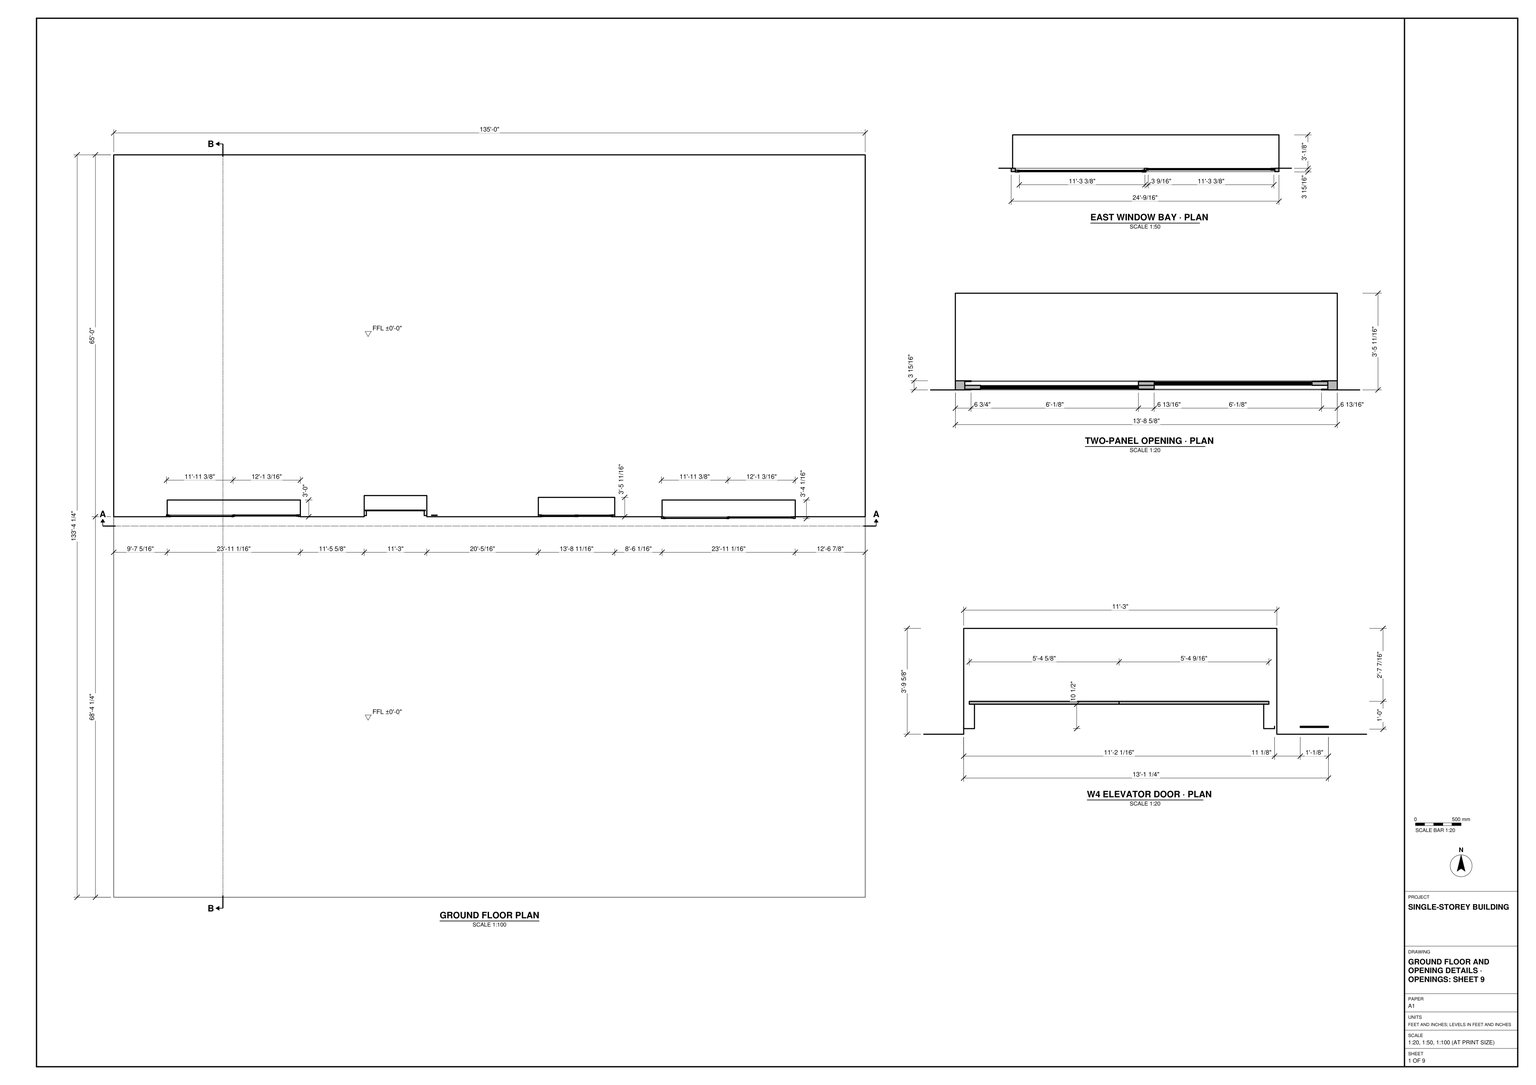
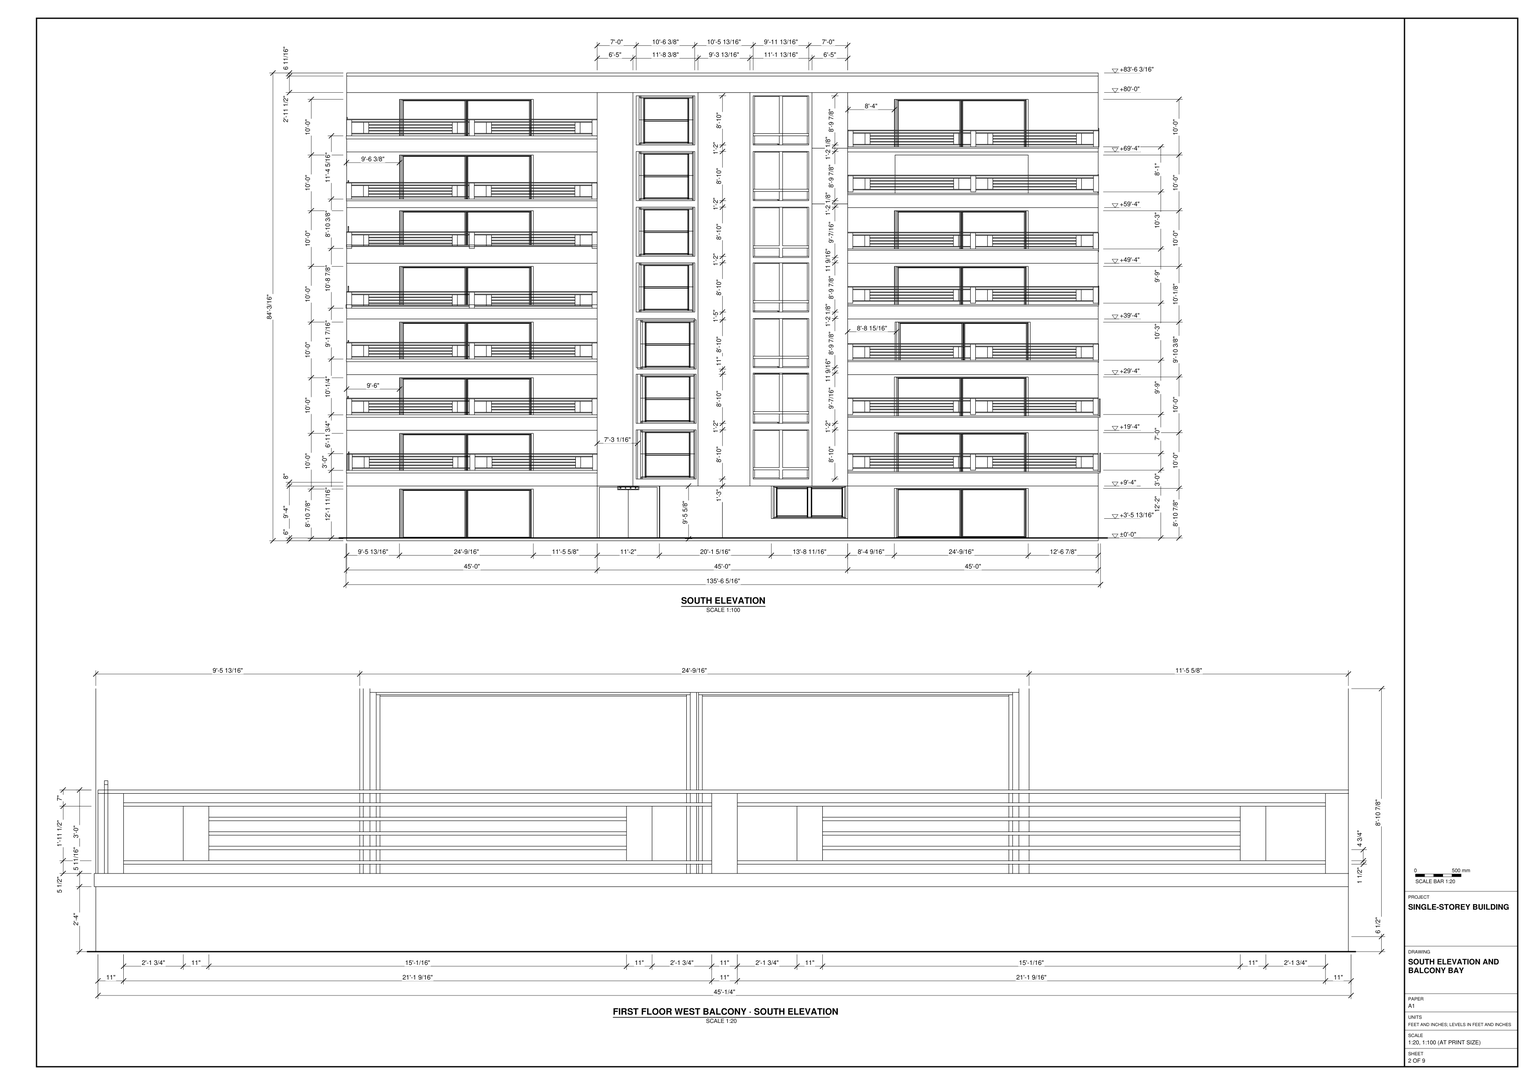
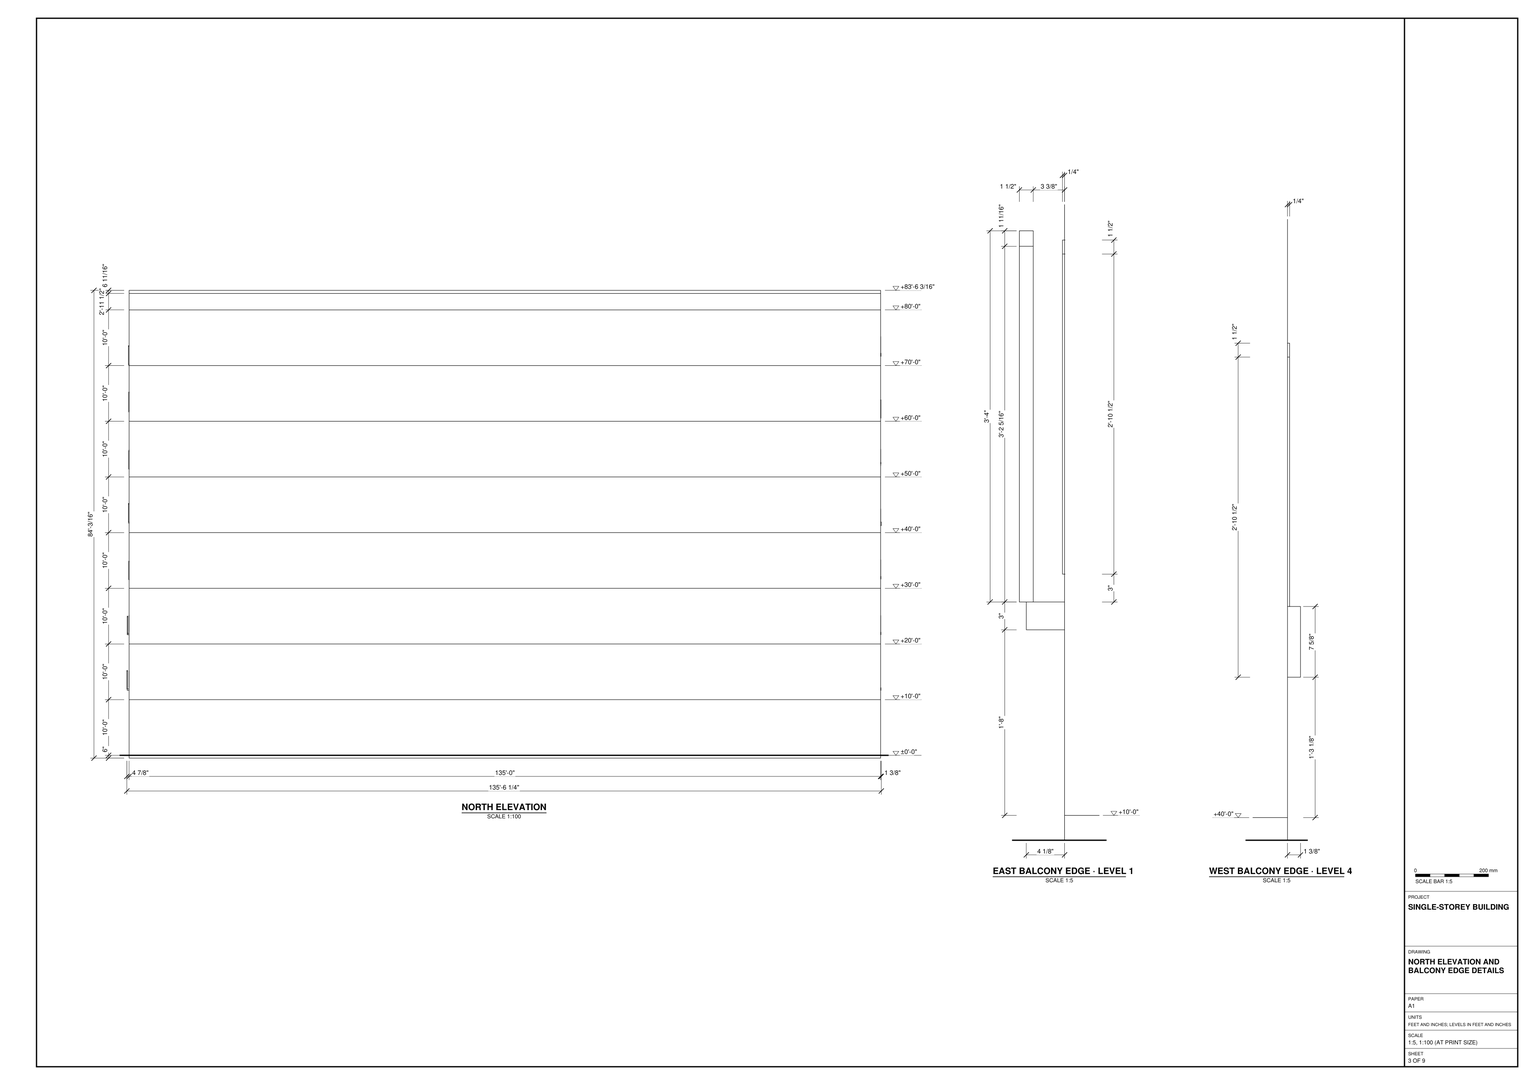
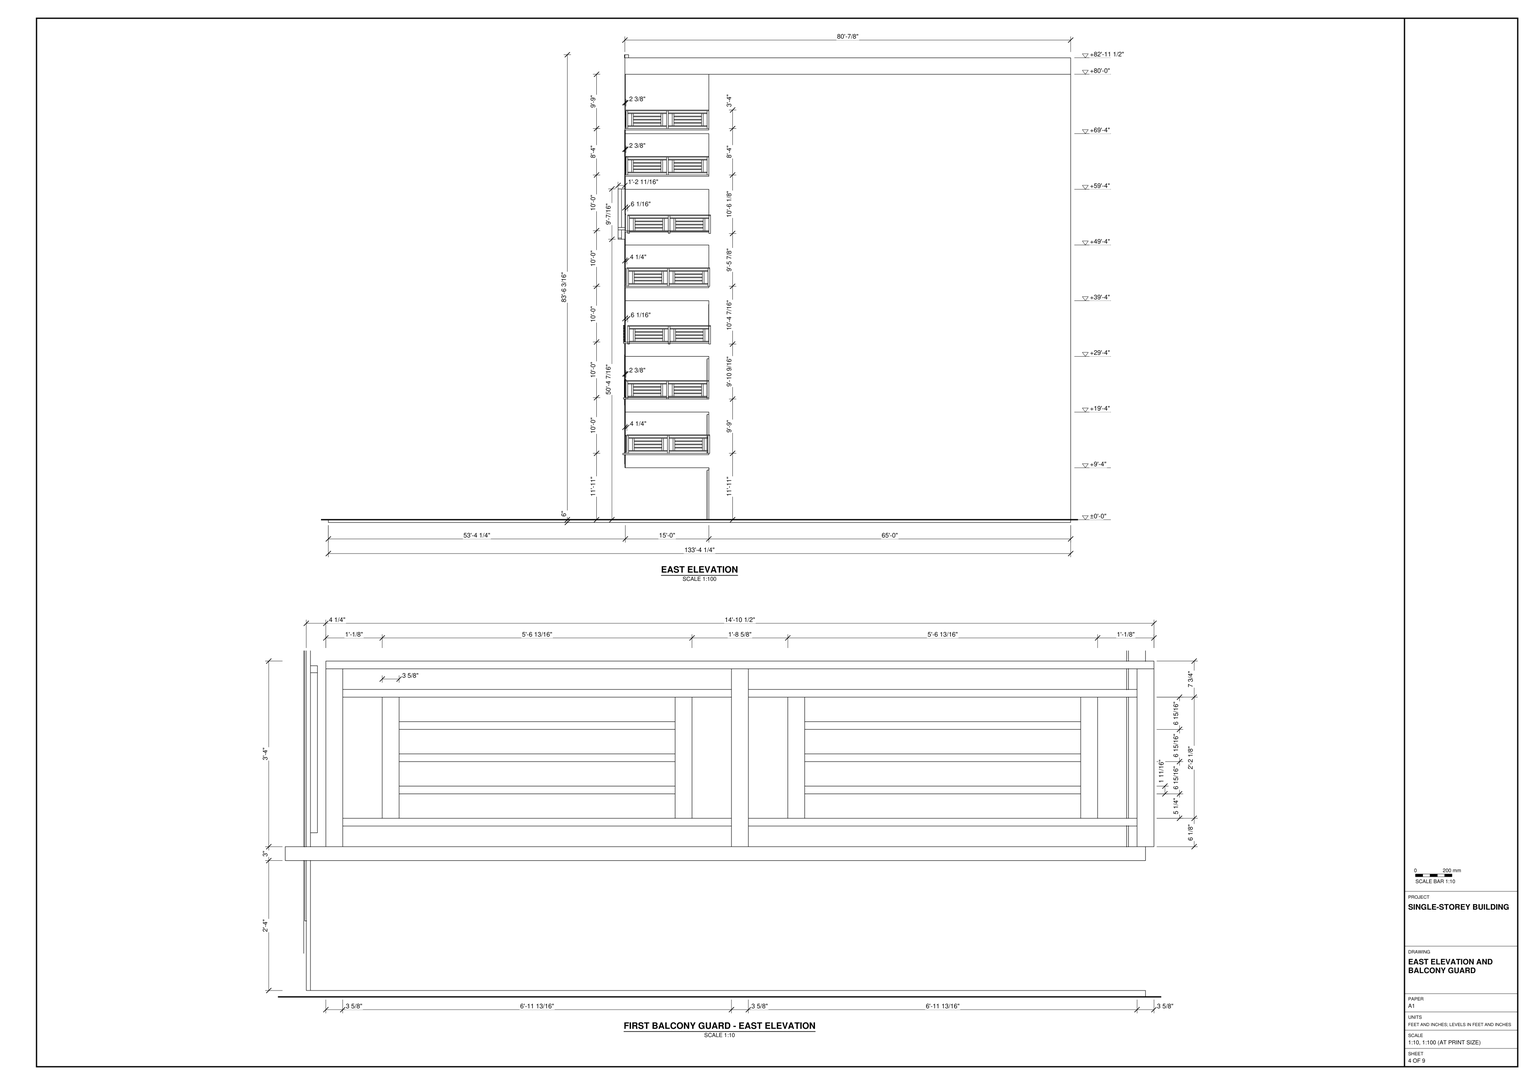
Build the building and its ground base in SketchUp from task_files/diagram_01.pdf. Work in feet and inches. Set the ground-floor finished level at ±0'-0". The overall model dimensions are 135'-6 1/4" along X, 133'-4 1/4" along Y and 84'-3/16" along Z. Use the plan to locate the south wall within the full depth of the base; the base continues south beyond the building.

Model the walls at the thicknesses drawn, with the floor slabs, balcony edges and flat roof following the elevations and sections. On the south face, place the wide outer openings behind the stacked balcony railings. Follow the balcony detail for the spacing of posts and horizontal rails. Keep the two narrower stacks of framed openings in the central bay distinct from the balcony bays. At ground level, use the opening plans to set the elevator door and the adjacent two-panel opening at their respective depths. Keep the north elevation plain, with the horizontal divisions shown.

Make shell elements such as walls, slabs and roof separate groups or components. Keep each furniture or joinery piece shown separate, and use components for repeated parts such as window units and railing sections. Any decor or loose items shown may use suitable library components. Save one SketchUp model as output_files/multi_storey_building_with_stacked_south_balconies.skp.

# SketchUp Ruby script. Lengths in inches.
U = 1.inch
M = Sketchup.active_model
def pt(a) = Geom::Point3d.new(a.map { |v| v * U })
def face(e, loops, mat)
  f = e.add_face(loops[0].map { |a| pt(a) })
  loops[1..].each { |l| e.add_face(l.map { |a| pt(a) }).erase! }
  f.material = f.back_material = mat if mat
  f
end
# faces: each face lists its corners as indices into pts; further lists are holes
def faces(e, pts, list, mat = nil) = list.each { |f| face(e, (f[0].is_a?(Array) ? f : [f]).map { |l| l.map { |i| pts[i] } }, mat) }
# xy, xz, yz: faces in a plane at the given z, y or x. An outline is a flat list of corners, or four numbers for a rectangle; further outlines are holes
def ring(l) = l.size == 4 ? [[l[0], l[1]], [l[2], l[1]], [l[2], l[3]], [l[0], l[3]]] : l.each_slice(2).to_a
def flat(e, list, mat, &to3) = list.each { |f| face(e, (f[0].is_a?(Array) ? f : [f]).map { |l| ring(l).map { |u, v| to3.(u, v) } }, mat) }
def xy(e, z, list, mat = nil) = flat(e, list, mat) { |x, y| [x, y, z] }
def xz(e, y, list, mat = nil) = flat(e, list, mat) { |x, z| [x, y, z] }
def yz(e, x, list, mat = nil) = flat(e, list, mat) { |y, z| [x, y, z] }
def lines(e, pts, list) = list.each { |a, b| e.add_line(pt(pts[a]), pt(pts[b])) }
# prism: a flat outline (further loops are holes) pulled along v
def prism(e, loops, v, mat = nil)
  f = face(e, loops, mat); d = Geom::Vector3d.new(v.map { |x| x * U })
  f.pushpull(f.normal.samedirection?(d) ? d.length : -d.length)
end
def box(e, o, s, mat = nil) = prism(e, [[o, [o[0] + s[0], o[1], o[2]], [o[0] + s[0], o[1] + s[1], o[2]], [o[0], o[1] + s[1], o[2]]]], [0, 0, s[2]], mat)
def at(x, y, z, deg = 0) = Geom::Transformation.translation(pt([x, y, z])) * Geom::Transformation.rotation(ORIGIN, Z_AXIS, deg.degrees)
def axes(o, x, y, z) = Geom::Transformation.new([*x, 0, *y, 0, *z, 0, *pt(o).to_a, 1])
def part(name) = M.definitions.add(name)
# library, detail: a bought-in or finely detailed component or shape, given as its bounding box
def library(name, o, s) = part(name).tap { |d| box(d.entities, o, s) }
def detail(e, o, s) = box(e.add_group.entities, o, s)
def put(e, d, t, mat = nil) = e.add_instance(d, t).tap { |i| i.material = mat if mat }
def group(e, t, mat = nil) = e.add_group.tap { |g| g.transformation = t; g.material = mat if mat }.entities
root = M.entities
M.materials.add("Glass_Tinted_Gray").color = [0, 0, 0]
M.materials["Glass_Tinted_Gray"].alpha = 0.125
M.materials.add("Painted Metal Railing").color = [35, 35, 35]
M.materials.add("[0043_SaddleBrown]").color = [139, 69, 19]
M.materials.add("[0047_Khaki]").color = [240, 230, 140]
M.materials.add("[0134_DimGray]").color = [105, 105, 105]
M.materials.add("[0135_DarkGray]").color = [81, 81, 81]
M.materials.add("[Mirror 02]").color = [229, 229, 229]
M.materials.add("[Terrazzo Light Blue]").color = [196, 214, 227]
c1 = library("Untitled",[0,0,0],[47.4375,3.75,63.125])
c2 = part("PENTEK_RP Fineline 50S_Sliding_DoorCase_E1")
box(c2.entities,[0,0,0],[1.51,3.66,99.27],"[0135_DarkGray]")
c3 = part("PENTEK_RP Fineline 50S_SlidingDooe_Case_E2")
box(c3.entities,[0,0,0],[96.25,3.66,1.51],"[0135_DarkGray]")
c4 = part("pentek_RP Fineline 50S_SlidingDoor_Case")
put(c4.entities,c2,at(97.76,0,0))
put(c4.entities,c3,at(1.51,0,0))
put(c4.entities,c2,at(0,0,0))
put(c4.entities,c3,at(1.51,0,97.76))
c5 = part("PENTEK_RP Fineline 50S_SlidingDoor_GlazingBead_2")
box(c5.entities,[0,0,0],[0.56,0.59,94.39],"[0135_DarkGray]")
c6 = part("PENTEK_RP Fineline 50S_SlidingDoor_Glass")
box(c6.entities,[0,0,0],[46.58,0.16,94.39],"Glass_Tinted_Gray")
c7 = part("PENTEK_RP Fineline 50S_SlidingDoor_GlazingBead")
box(c7.entities,[0,0,0],[45.47,0.59,0.56],"[0135_DarkGray]")
c8 = part("PENTEK_RP Fineline 50S_SlidingDoor_Leaf_E1")
xy(c8.entities,0,[[0,0,0.93,1.97],[0.93,1.57,1.49,1.97]],"[0135_DarkGray]")
xy(c8.entities,96.25,[[0,0,0.93,0,0.93,1.57,1.49,1.57,1.49,1.97,0,1.97]],"[0135_DarkGray]")
xz(c8.entities,0,[[0,0,0.93,96.25]],"[0135_DarkGray]")
xz(c8.entities,1.57,[[0.93,0,1.49,95.32],[0.93,95.32,1.49,96.25]],"[0135_DarkGray]")
xz(c8.entities,1.97,[[0,0,1.49,96.25]],"[0135_DarkGray]")
yz(c8.entities,0,[[0,0,1.97,96.25]],"[0135_DarkGray]")
yz(c8.entities,0.93,[[0,0,1.57,0.93],[0,0.93,1.57,95.32],[0,95.32,1.57,96.25]],"[0135_DarkGray]")
yz(c8.entities,1.49,[[1.57,0,1.97,95.32],[1.57,95.32,1.97,96.25]],"[0135_DarkGray]")
c9 = part("PENTEK_RP Fineline 50S_SlidingDoor_Leaf_E2")
xy(c9.entities,0,[[0,0,0,1.57,0.56,1.57,0.56,1.97,46.02,1.97,46.02,1.57,46.58,1.57,46.58,0]],"[0135_DarkGray]")
xy(c9.entities,0.93,[[0,0,46.58,1.57]],"[0135_DarkGray]")
xy(c9.entities,1.49,[[0.56,1.57,46.02,1.97]],"[0135_DarkGray]")
xz(c9.entities,0,[[0,0,46.58,0.93]],"[0135_DarkGray]")
xz(c9.entities,1.57,[[0,0,0.56,0.93],[46.02,0,46.58,0.93],[0.56,0.93,46.02,1.49]],"[0135_DarkGray]")
xz(c9.entities,1.97,[[0.56,0,46.02,1.49]],"[0135_DarkGray]")
yz(c9.entities,0,[[0,0,1.57,0.93]],"[0135_DarkGray]")
yz(c9.entities,0.56,[[1.57,0,1.97,0.93],[1.57,0.93,1.97,1.49]],"[0135_DarkGray]")
yz(c9.entities,46.02,[[1.57,0,1.97,0.93],[1.57,0.93,1.97,1.49]],"[0135_DarkGray]")
yz(c9.entities,46.58,[[0,0,1.57,0.93]],"[0135_DarkGray]")
c10 = part("PENTEK_RP Fineline S_SlidingDoor_Leaf1")
put(c10.entities,c5,at(0.93,0,0.93))
put(c10.entities,c5,at(46.96,0,0.93))
put(c10.entities,c6,at(1.49,1.42,0.93))
put(c10.entities,c7,at(1.49,0,0.93))
put(c10.entities,c6,at(1.49,0.59,0.93),"[Terrazzo Light Blue]")
put(c10.entities,c8,at(0,0,0))
put(c10.entities,c8,axes([48.44,0,0],[-1,0,0],[0,1,0],[0,0,1]))
put(c10.entities,c9,axes([0.93,0,96.25],[1,0,0],[0,1,0],[0,0,-1]))
put(c10.entities,c9,at(0.93,0,0))
put(c10.entities,c7,at(1.49,0,94.77))
c11 = part("PENTEK_RP Fineline 50S_SlidingDoor_Leaf2")
put(c11.entities,c6,at(1.49,1.42,0.93))
put(c11.entities,c7,at(1.49,0,94.77))
put(c11.entities,c5,at(46.96,0,0.93))
put(c11.entities,c6,at(1.49,0.59,0.93),"[Mirror 02]")
put(c11.entities,c5,at(0.93,0,0.93))
put(c11.entities,c8,at(0,0,0))
put(c11.entities,c8,axes([48.44,0,0],[-1,0,0],[0,1,0],[0,0,1]))
put(c11.entities,c7,at(1.49,0,0.93))
put(c11.entities,c9,axes([0.93,0,96.25],[1,0,0],[0,1,0],[0,0,-1]))
put(c11.entities,c9,at(0.93,0,0))
c12 = part("PENTEK - Slimmest Steel Sliding Door / Window\#1")
put(c12.entities,c4,at(0,-1.88,-0.09))
put(c12.entities,c10,at(1.51,-2.27,1.42))
put(c12.entities,c11,at(49.32,-0.3,1.42))
c13 = library("Elevator_Door[140]",[-13.125,-2.71,-1.46],[68.625,12,93.74])
c14 = part("Post")
box(c14.entities,[-0.75,-0.75,0],[1.5,1.5,34.5],"Painted Metal Railing")
c15 = part("Group43\#1")
box(c15.entities,[-0.75,0,0],[1.5,73.5,1.5],"Painted Metal Railing")
c16 = part("Group46\#1")
box(c16.entities,[-0.75,0.75,0],[1.5,34.5,1.5],"Painted Metal Railing")
c17 = part("Group49\#1")
box(c17.entities,[-0.75,0.75,0],[1.5,34.5,1.5],"Painted Metal Railing")
c18 = part("Group52\#1")
box(c18.entities,[-0.75,0.75,0],[1.5,34.5,1.5],"Painted Metal Railing")
c19 = part("Group55\#1")
box(c19.entities,[-0.75,0.75,0],[1.5,34.5,1.5],"Painted Metal Railing")
c20 = part("Inner Post")
box(c20.entities,[-0.75,-0.75,0],[1.5,1.5,23.5],"Painted Metal Railing")
c21 = part("Group59\#1")
box(c21.entities,[-0.75,0.75,0],[1.5,24.5,1.5],"Painted Metal Railing")
c22 = part("Group62\#1")
box(c22.entities,[-0.75,0.75,0],[1.5,24.5,1.5],"Painted Metal Railing")
c23 = part("Group65\#1")
box(c23.entities,[-0.75,0.75,0],[1.5,24.5,1.5],"Painted Metal Railing")
c24 = part("Inner Posts and Rails\#2")
put(c24.entities,c20,at(0,0,0,90))
put(c24.entities,c20,at(0,26,0,90))
put(c24.entities,c21,at(0,0,4.75))
put(c24.entities,c22,at(0,0,11))
put(c24.entities,c23,at(0,0,17.25))
c25 = part("Group69\#1")
box(c25.entities,[-0.75,0.75,0],[1.5,24.5,1.5],"Painted Metal Railing")
c26 = part("Group72\#1")
box(c26.entities,[-0.75,0.75,0],[1.5,24.5,1.5],"Painted Metal Railing")
c27 = part("Group75\#1")
box(c27.entities,[-0.75,0.75,0],[1.5,24.5,1.5],"Painted Metal Railing")
c28 = part("Inner Posts and Rails\#3")
put(c28.entities,c20,at(0,0,0,90))
put(c28.entities,c20,at(0,26,0,90))
put(c28.entities,c25,at(0,0,4.75))
put(c28.entities,c26,at(0,0,11))
put(c28.entities,c27,at(0,0,17.25))
c29 = part("Railing Assembly 14\#1")
put(c29.entities,c14,at(0,0,0))
put(c29.entities,c14,at(36,0,0))
put(c29.entities,c14,at(72,0,0))
put(c29.entities,c15,at(-0.75,0,34.5,-90))
put(c29.entities,c16,at(0,0,4,-90))
put(c29.entities,c17,at(36,0,4,-90))
put(c29.entities,c18,at(0,0,29,-90))
put(c29.entities,c19,at(36,0,29,-90))
put(c29.entities,c24,at(5,0,5.5,-90))
put(c29.entities,c28,at(41,0,5.5,-90))
c30 = part("Railing Assembly 14\#2")
put(c30.entities,c14,at(0,0,0))
put(c30.entities,c14,at(36,0,0))
put(c30.entities,c14,at(72,0,0))
put(c30.entities,c15,at(-0.75,0,34.5,-90))
put(c30.entities,c16,at(0,0,4,-90))
put(c30.entities,c17,at(36,0,4,-90))
put(c30.entities,c18,at(0,0,29,-90))
put(c30.entities,c19,at(36,0,29,-90))
put(c30.entities,c24,at(5,0,5.5,-90))
put(c30.entities,c28,at(41,0,5.5,-90))
c31 = library("Group\#21",[0,0,0],[47.24,3.9375,39.37])
c32 = library("Group\#22",[0,0,0],[23.62,3.9375,39.37])
xy(root,-6,[[1.4,0,1621.4,1600.25]])
xy(root,0,[[1.4,0,1621.4,0,1621.4,820.25,1470.54,820.25,1470.54,856.25,1183.49,856.25,1183.49,820.25,676.4,820.25,676.4,865.875,541.4,865.875,541.4,820.25,403.75,820.25,403.75,856.25,116.7,856.25,116.7,820.25,1.4,820.25],[1.4,820.25,116.7,820.25,116.7,856.25,403.75,856.25,403.75,820.25,541.4,820.25,541.4,865.875,676.4,865.875,676.4,820.25,1183.49,820.25,1183.49,856.25,1470.54,856.25,1470.54,820.25,1621.4,820.25,1621.4,1600.25,1.4,1600.25]])
xy(root,41.8125,[[916.73,820.25,1081.4,861.9375]])
xy(root,105.375,[[116.7,820.25,403.75,856.25],[1183.49,820.25,1470.54,856.25]])
xy(root,112,[[618.42,639.35,618.42,640.25,1.4,640.25,1.4,820.25,541.4,820.25,541.4,865.875,676.4,865.875,676.4,820.25,916.73,820.25,916.73,861.9375,1081.4,861.9375,1081.4,820.25,1621.4,820.25,1621.4,640.25,1004.4,640.25,1004.4,639.35,870.61,639.35,870.61,640.25,870.58,640.25,870.58,642.9375,758.8,642.9375,758.8,639.35]])
xy(root,120,[[870.58,639.35,870.61,640.25],[7.4,646.25,541.4,646.25,541.4,820.25,403.75,820.25,403.75,856.25,116.7,856.25,116.7,820.25,7.4,820.25],[1081.4,648.25,1613.4,648.25,1613.4,820.25,1470.54,820.25,1470.54,856.25,1183.49,856.25,1183.49,820.25,1081.4,820.25]])
xy(root,127,[[625.42,639.35,751.8,651.25],[877.58,639.35,997.4,651.25]])
xy(root,140,[[1081.4,634.8125,1621.4,640.25],[1621.4,634.8125,1625.52,820.25],[0.7,639.55,541.4,640.25],[0.7,640.25,1.4,820.25],[1.4,640.25,1.4,820.25,7.4,820.25,7.4,646.25,541.4,646.25,541.4,640.25],
  [1081.4,640.25,1081.4,648.25,1613.4,648.25,1613.4,820.25,1621.4,820.25,1621.4,640.25]])
xy(root,143,[[1081.4,634.8125,1625.52,634.8125,1625.52,820.25,1613.4,820.25,1613.4,648.25,1081.4,648.25]])
xy(root,145.6875,[[0.7,639.55,541.4,639.55,541.4,646.25,7.4,646.25,7.4,820.25,0.7,820.25]])
xy(root,225.375,[[116.7,820.25,403.75,856.25],[1183.49,820.25,1470.54,856.25]])
xy(root,232,[[1.4,640.25,541.4,820.25],[1081.4,640.25,1621.4,820.25]])
xy(root,233,[[625.42,639.35,751.8,651.25],[877.58,639.35,997.4,651.25]])
xy(root,240,[[7.4,646.25,541.4,646.25,541.4,820.25,403.75,820.25,403.75,856.25,116.7,856.25,116.7,820.25,7.4,820.25],[1081.4,648.25,1613.4,648.25,1613.4,820.25,1470.54,820.25,1470.54,856.25,1183.49,856.25,1183.49,820.25,1081.4,820.25]])
xy(root,247,[[625.42,639.35,751.8,651.25],[877.58,639.35,997.4,651.25]])
xy(root,260,[[1081.4,636.125,1621.4,640.25],[1621.4,636.125,1625.52,820.25],[0.7,639.55,1.4,820.25],[1.4,639.55,541.4,640.25],[1.4,640.25,1.4,820.25,7.4,820.25,7.4,646.25,541.4,646.25,541.4,640.25],
  [1081.4,640.25,1081.4,648.25,1613.4,648.25,1613.4,820.25,1621.4,820.25,1621.4,640.25]])
xy(root,263,[[1081.4,636.125,1625.52,636.125,1625.52,820.25,1613.4,820.25,1613.4,648.25,1081.4,648.25]])
xy(root,265.4375,[[0.7,639.55,541.4,639.55,541.4,646.25,7.4,646.25,7.4,820.25,0.7,820.25]])
xy(root,345.375,[[116.7,820.25,403.75,856.25],[1183.49,820.25,1470.54,856.25]])
xy(root,352,[[1.4,640.25,541.4,820.25],[1081.4,640.25,1621.4,820.25]])
xy(root,353,[[625.42,639.35,751.8,651.25],[877.58,639.35,997.4,651.25]])
xy(root,360,[[7.4,646.25,541.4,646.25,541.4,820.25,403.75,820.25,403.75,856.25,116.7,856.25,116.7,820.25,7.4,820.25],[1081.4,648.25,1613.4,648.25,1613.4,820.25,1470.54,820.25,1470.54,856.25,1183.49,856.25,1183.49,820.25,1081.4,820.25]])
xy(root,367,[[625.42,639.35,751.8,651.25],[877.58,639.35,997.4,651.25]])
xy(root,380,[[1081.4,636.125,1621.4,640.25],[1621.4,636.125,1622.2,820.25],[0.7,639.55,541.4,640.25],[0.7,640.25,1.4,820.25],[1.4,640.25,1.4,820.25,7.4,820.25,7.4,646.25,541.4,646.25,541.4,640.25],
  [1081.4,640.25,1081.4,648.25,1613.4,648.25,1613.4,820.25,1621.4,820.25,1621.4,640.25]])
xy(root,383,[[1081.4,636.125,1622.2,636.125,1622.2,820.25,1613.4,820.25,1613.4,648.25,1081.4,648.25]])
xy(root,385.6875,[[0.7,639.55,541.4,639.55,541.4,646.25,7.4,646.25,7.4,820.25,0.7,820.25]])
xy(root,465.375,[[116.7,820.25,403.75,856.25],[1183.49,820.25,1470.54,856.25]])
xy(root,472,[[1.4,640.25,541.4,820.25],[1081.4,640.25,1621.4,820.25]])
xy(root,473,[[625.42,639.35,751.8,651.25],[877.58,639.35,997.4,651.25]])
xy(root,480,[[7.4,646.25,541.4,646.25,541.4,820.25,403.75,820.25,403.75,856.25,116.7,856.25,116.7,820.25,7.4,820.25],[1081.4,648.25,1613.4,648.25,1613.4,820.25,1470.54,820.25,1470.54,856.25,1183.49,856.25,1183.49,820.25,1081.4,820.25]])
xy(root,487,[[625.42,639.35,751.8,651.25],[877.58,639.35,997.4,651.25]])
xy(root,495.125,[[0,638.85,541.4,640.25],[0,640.25,1.4,820.25],[1.4,640.25,1.4,820.25,7.4,820.25,7.4,646.25,541.4,646.25,541.4,640.25]])
xy(root,500,[[1081.4,639.45,1621.4,640.25],[1621.4,639.45,1622.2,820.25],[1081.4,640.25,1081.4,648.25,1613.4,648.25,1613.4,820.25,1621.4,820.25,1621.4,640.25]])
xy(root,502.75,[[0,638.85,541.4,638.85,541.4,646.25,7.4,646.25,7.4,820.25,0,820.25]])
xy(root,503,[[1081.4,639.45,1622.2,639.45,1622.2,820.25,1613.4,820.25,1613.4,648.25,1081.4,648.25]])
xy(root,585.375,[[116.7,820.25,403.75,856.25],[1183.49,820.25,1470.54,856.25]])
xy(root,592,[[1.4,640.25,541.4,820.25],[1081.4,640.25,1621.4,820.25]])
xy(root,593,[[625.42,639.35,751.8,651.25],[877.58,639.35,997.4,651.25]])
xy(root,600,[[7.4,646.25,541.4,646.25,541.4,820.25,403.75,820.25,403.75,856.25,116.7,856.25,116.7,820.25,7.4,820.25],[1081.4,648.25,1613.4,648.25,1613.4,820.25,1470.54,820.25,1470.54,856.25,1183.49,856.25,1183.49,820.25,1081.4,820.25]])
xy(root,607,[[625.42,639.35,751.8,651.25],[877.58,639.35,997.4,651.25]])
xy(root,620,[[1081.4,639.45,1621.4,640.25],[1621.4,639.45,1622.2,820.25],[1081.4,640.25,1081.4,648.25,1613.4,648.25,1613.4,820.25,1621.4,820.25,1621.4,640.25]])
xy(root,623,[[1081.4,639.45,1622.2,639.45,1622.2,820.25,1613.4,820.25,1613.4,648.25,1081.4,648.25]])
xy(root,628,[[0.7,639.55,541.4,640.25],[0.7,640.25,1.4,820.25],[1.4,640.25,1.4,820.25,7.4,820.25,7.4,646.25,541.4,646.25,541.4,640.25]])
xy(root,631.625,[[0.7,639.55,541.4,639.55,541.4,646.25,7.4,646.25,7.4,820.25,0.7,820.25]])
xy(root,705.375,[[116.7,820.25,403.75,856.25],[1183.49,820.25,1470.54,856.25]])
xy(root,712,[[1.4,640.25,541.4,820.25],[1081.4,640.25,1621.4,820.25]])
xy(root,713,[[625.42,639.35,751.8,651.25],[877.58,639.35,997.4,651.25]])
xy(root,720,[[7.4,646.25,541.4,646.25,541.4,820.25,403.75,820.25,403.75,856.25,116.7,856.25,116.7,820.25,7.4,820.25],[1081.4,648.25,1613.4,648.25,1613.4,820.25,1470.54,820.25,1470.54,856.25,1183.49,856.25,1183.49,820.25,1081.4,820.25]])
xy(root,726.6875,[[0.8,639.65,541.4,640.25],[0.8,640.25,1.4,820.25],[1.4,640.25,1.4,820.25,7.4,820.25,7.4,646.25,541.4,646.25,541.4,640.25]])
xy(root,727,[[625.42,639.35,751.8,651.25],[877.58,639.35,997.4,651.25]])
xy(root,730.375,[[0.8,639.65,541.4,639.65,541.4,646.25,7.4,646.25,7.4,820.25,0.8,820.25]],"[0043_SaddleBrown]")
xy(root,740,[[1081.4,639.45,1621.4,640.25],[1621.4,639.45,1622.2,820.25],[1081.4,640.25,1081.4,648.25,1613.4,648.25,1613.4,820.25,1621.4,820.25,1621.4,640.25]])
xy(root,743,[[1081.4,639.45,1622.2,639.45,1622.2,820.25,1613.4,820.25,1613.4,648.25,1081.4,648.25]])
xy(root,825.375,[[116.7,820.25,403.75,856.25],[1183.49,820.25,1470.54,856.25]])
xy(root,832,[[1.4,640.25,541.4,820.25],[1081.4,640.25,1621.4,820.25]])
xy(root,833,[[625.42,639.35,751.8,651.25],[877.58,639.35,997.4,651.25]])
xy(root,840,[[1081.4,639.45,1621.4,640.25],[1621.4,639.45,1622.2,820.25],[1081.4,640.25,1081.4,648.25,1613.4,648.25,1613.4,820.25,1621.4,820.25,1621.4,640.25],[7.4,646.25,541.4,646.25,541.4,820.25,403.75,820.25,403.75,856.25,116.7,856.25,116.7,820.25,7.4,820.25],[1081.4,648.25,1613.4,648.25,1613.4,820.25,1470.54,820.25,1470.54,856.25,1183.49,856.25,1183.49,820.25,1081.4,820.25]])
xy(root,843,[[1081.4,639.45,1622.2,639.45,1622.2,820.25,1613.4,820.25,1613.4,648.25,1081.4,648.25]])
xy(root,847,[[625.42,639.35,751.8,651.25],[877.58,639.35,997.4,651.25]])
xy(root,860,[[0.6,639.45,1.4,640.25],[1.4,639.45,541.4,640.25],[0.6,640.25,1.4,820.25],[1.4,640.25,1.4,820.25,7.4,820.25,7.4,646.25,541.4,646.25,541.4,640.25]])
xy(root,866.6875,[[0.6,639.45,541.4,639.45,541.4,646.25,7.4,646.25,7.4,820.25,0.6,820.25]])
xy(root,945.375,[[116.7,820.25,403.75,856.25],[1183.49,820.25,1470.54,856.25]])
xy(root,953,[[625.42,639.35,751.8,651.25],[877.58,639.35,997.4,651.25]])
xy(root,960,[[1.4,639.35,541.4,820.25],[618.42,639.35,618.42,640.25,541.4,640.25,541.4,820.25,1.4,820.25,1.4,1600.25,1621.4,1600.25,1621.4,820.25,1081.4,820.25,1081.4,640.25,1004.4,640.25,1004.4,639.35,870.58,639.35,870.58,642.9375,758.8,642.9375,758.8,639.35],[541.4,639.35,618.42,640.25],[758.8,639.35,870.58,642.9375],[1004.4,639.35,1081.4,640.25],
  [1081.4,639.35,1621.4,820.25]])
xy(root,995.5,[[1.4,639.35,1621.4,647.35],[1.4,647.35,1621.4,1600.25]])
xy(root,995.5,[[1.4,638.45,1621.4,639.35]],"[0043_SaddleBrown]")
xy(root,1002.1875,[[1.4,638.45,1621.4,647.35]])
xz(root,0,[[1.4,-6,1621.4,0]])
xz(root,634.8125,[[1081.4,140,1625.52,143]])
xz(root,636.125,[[1081.4,260,1625.52,263],[1081.4,380,1622.2,383]])
xz(root,638.45,[[1.4,995.5,1621.4,1002.1875]],"[0043_SaddleBrown]")
xz(root,638.85,[[0,495.125,541.4,502.75]],"[0043_SaddleBrown]")
xz(root,639.35,[[1.4,960,1621.4,995.5]])
xz(root,639.35,[[[618.42,112,758.8,960],[625.42,847,751.8,953],[625.42,607,751.8,713],[625.42,367,751.8,473],[625.42,127,751.8,233],[625.42,247,751.8,353],[625.42,487,751.8,593],[625.42,727,751.8,833]],[[870.61,112,1004.4,112,1004.4,960,870.58,960,870.58,120,870.61,120],[877.58,247,997.4,353],[877.58,847,997.4,953],[877.58,607,997.4,713],[877.58,127,997.4,233],[877.58,487,997.4,593],[877.58,727,997.4,833],[877.58,367,997.4,473]]],"[0134_DimGray]")
xz(root,639.45,[[1081.4,500,1622.2,503],[1081.4,620,1622.2,623],[1081.4,740,1622.2,743],[1081.4,840,1622.2,843],[0.6,860,541.4,866.6875]])
xz(root,639.55,[[0.7,140,541.4,145.6875]])
xz(root,639.55,[[0.7,260,541.4,265.4375],[0.7,380,541.4,385.6875],[0.7,628,541.4,631.625]],"[0043_SaddleBrown]")
xz(root,639.65,[[0.8,726.6875,541.4,730.375]],"[0043_SaddleBrown]")
xz(root,640.25,[[1.4,112,541.4,140],[870.58,112,870.61,120],[1081.4,112,1621.4,140],[1.4,232,541.4,260],[1081.4,232,1621.4,260],
  [1.4,352,541.4,380],[1081.4,352,1621.4,380],[1.4,472,541.4,495.125],[1081.4,472,1621.4,500],[1.4,592,541.4,628],
  [1081.4,592,1621.4,620],[1.4,712,541.4,726.6875],[1081.4,712,1621.4,740],[1.4,832,541.4,860],[1081.4,832,1621.4,840]])
xz(root,640.25,[[541.4,112,618.42,960],[1004.4,112,1081.4,720],[1004.4,720,1081.4,840],[1004.4,840,1081.4,960]],"[0134_DimGray]")
xz(root,642.9375,[[758.8,112,870.58,960]],"[0134_DimGray]")
xz(root,646.25,[[7.4,120,541.4,140],[7.4,140,541.4,145.6875],[7.4,240,541.4,260],[7.4,260,541.4,265.4375],[7.4,360,541.4,380],
  [7.4,380,541.4,385.6875],[7.4,480,541.4,495.125],[7.4,495.125,541.4,502.75],[7.4,600,541.4,628],[7.4,628,541.4,631.625],
  [7.4,720,541.4,726.6875],[7.4,726.6875,541.4,730.375],[7.4,840,541.4,860],[7.4,860,541.4,866.6875]])
xz(root,647.35,[[1.4,995.5,1621.4,1002.1875]])
xz(root,648.25,[[1081.4,120,1613.4,140],[1081.4,140,1613.4,143],[1081.4,240,1613.4,260],[1081.4,260,1613.4,263],[1081.4,360,1613.4,380],
  [1081.4,380,1613.4,383],[1081.4,480,1613.4,500],[1081.4,500,1613.4,503],[1081.4,600,1613.4,620],[1081.4,620,1613.4,623],
  [1081.4,720,1613.4,740],[1081.4,740,1613.4,743],[1081.4,840,1613.4,843]])
xz(root,651.25,[[625.42,127,751.8,233],[877.58,127,997.4,233],[625.42,247,751.8,353],[877.58,247,997.4,353],[625.42,367,751.8,473],
  [877.58,367,997.4,473],[625.42,487,751.8,593],[877.58,487,997.4,593],[625.42,607,751.8,713],[877.58,607,997.4,713],
  [625.42,727,751.8,833],[877.58,727,997.4,833],[625.42,847,751.8,953],[877.58,847,997.4,953]])
xz(root,820.25,[[0.7,140,1.4,145.6875],[1.4,140,7.4,145.6875],[1613.4,140,1621.4,143],[1621.4,140,1625.52,143],[0.7,260,1.4,265.4375],
  [1.4,260,7.4,265.4375],[1613.4,260,1621.4,263],[1621.4,260,1625.52,263],[1.4,360,7.4,380],[0.7,380,1.4,385.6875],
  [1.4,380,7.4,385.6875],[1613.4,380,1621.4,383],[1621.4,380,1622.2,383],[0,495.125,1.4,502.75],[1.4,495.125,7.4,502.75],
  [1613.4,500,1621.4,503],[1621.4,500,1622.2,503],[1613.4,620,1621.4,623],[1621.4,620,1622.2,623],[0.7,628,1.4,631.625],
  [1.4,628,7.4,631.625],[1.4,720,7.4,726.6875],[0.8,726.6875,1.4,730.375],[1.4,726.6875,7.4,730.375],[1613.4,740,1621.4,743],
  [1621.4,740,1622.2,743],[1613.4,840,1621.4,843],[1621.4,840,1622.2,843],[0.6,860,1.4,866.6875],[1.4,860,7.4,866.6875]])
xz(root,820.25,[[1.4,0,116.7,0,116.7,105.375,403.75,105.375,403.75,0,541.4,0,541.4,112,1.4,112],[676.4,0,811.4,112],[811.4,0,1081.4,0,1081.4,41.8125,916.73,41.8125,916.73,112,811.4,112],[1081.4,0,1183.49,0,1183.49,105.375,1470.54,105.375,1470.54,0,1621.4,0,1621.4,112,1081.4,112],[7.4,120,116.7,120,116.7,225.375,403.75,225.375,403.75,120,541.4,120,541.4,232,1.4,232,1.4,145.6875,7.4,145.6875],
  [1081.4,120,1183.49,120,1183.49,225.375,1470.54,225.375,1470.54,120,1613.4,120,1613.4,143,1621.4,143,1621.4,232,1081.4,232],[7.4,240,116.7,240,116.7,345.375,403.75,345.375,403.75,240,541.4,240,541.4,352,1.4,352,1.4,265.4375,7.4,265.4375],[1081.4,240,1183.49,240,1183.49,345.375,1470.54,345.375,1470.54,240,1613.4,240,1613.4,263,1621.4,263,1621.4,352,1081.4,352],[7.4,360,116.7,360,116.7,465.375,403.75,465.375,403.75,360,541.4,360,541.4,472,1.4,472,1.4,385.6875,7.4,385.6875],[1081.4,360,1183.49,360,1183.49,465.375,1470.54,465.375,1470.54,360,1613.4,360,1613.4,383,1621.4,383,1621.4,472,1081.4,472],
  [7.4,480,116.7,480,116.7,585.375,403.75,585.375,403.75,480,541.4,480,541.4,592,1.4,592,1.4,502.75,7.4,502.75],[1081.4,480,1183.49,480,1183.49,585.375,1470.54,585.375,1470.54,480,1613.4,480,1613.4,503,1621.4,503,1621.4,592,1081.4,592],[7.4,600,116.7,600,116.7,705.375,403.75,705.375,403.75,600,541.4,600,541.4,712,1.4,712,1.4,631.625,7.4,631.625],[1081.4,600,1183.49,600,1183.49,705.375,1470.54,705.375,1470.54,600,1613.4,600,1613.4,623,1621.4,623,1621.4,712,1081.4,712],[7.4,720,116.7,720,116.7,825.375,403.75,825.375,403.75,720,541.4,720,541.4,832,1.4,832,1.4,730.375,7.4,730.375],
  [1081.4,720,1183.49,720,1183.49,825.375,1470.54,825.375,1470.54,720,1613.4,720,1613.4,743,1621.4,743,1621.4,832,1081.4,832],[7.4,840,116.7,840,116.7,945.375,403.75,945.375,403.75,840,541.4,840,541.4,960,1.4,960,1.4,866.6875,7.4,866.6875],[1081.4,840,1183.49,840,1183.49,945.375,1470.54,945.375,1470.54,840,1613.4,840,1613.4,843,1621.4,843,1621.4,960,1081.4,960]],"[0047_Khaki]")
xz(root,856.25,[[116.7,0,403.75,105.375],[1183.49,0,1470.54,105.375],[116.7,120,403.75,225.375],[1183.49,120,1470.54,225.375],[116.7,240,403.75,345.375],
  [1183.49,240,1470.54,345.375],[116.7,360,403.75,465.375],[1183.49,360,1470.54,465.375],[116.7,480,403.75,585.375],[1183.49,480,1470.54,585.375],
  [116.7,600,403.75,705.375],[1183.49,600,1470.54,705.375],[116.7,720,403.75,825.375],[1183.49,720,1470.54,825.375],[116.7,840,403.75,945.375],
  [1183.49,840,1470.54,945.375]])
xz(root,861.9375,[[916.73,41.8125,1081.4,112]])
xz(root,865.875,[[541.4,0,676.4,112]])
xz(root,1600.25,[[1.4,-6,1621.4,0],[1.4,0,1621.4,120],[1.4,120,1621.4,240],[1.4,240,1621.4,360],[1.4,360,1621.4,480],
  [1.4,480,1621.4,600],[1.4,600,1621.4,720],[1.4,720,1621.4,840],[1.4,840,1621.4,960],[1.4,960,1621.4,995.5]])
yz(root,0,[[638.85,495.125,820.25,502.75]],"[0043_SaddleBrown]")
yz(root,0.6,[[639.45,860,820.25,866.6875]])
yz(root,0.7,[[639.55,140,820.25,145.6875]])
yz(root,0.7,[[639.55,260,820.25,265.4375],[639.55,380,820.25,385.6875],[639.55,628,820.25,631.625]],"[0043_SaddleBrown]")
yz(root,0.8,[[639.65,726.6875,820.25,730.375]],"[0043_SaddleBrown]")
yz(root,1.4,[[0,-6,1600.25,0],[820.25,0,820.25,112,640.25,112,640.25,140,820.25,140,820.25,232,640.25,232,640.25,260,820.25,260,820.25,352,640.25,352,640.25,380,820.25,380,820.25,472,640.25,472,640.25,495.125,820.25,495.125,820.25,592,640.25,592,640.25,628,820.25,628,820.25,712,640.25,712,640.25,726.6875,820.25,726.6875,820.25,832,640.25,832,640.25,860,820.25,860,820.25,960,1600.25,960,1600.25,0],[639.35,960,1600.25,995.5]])
yz(root,1.4,[[638.45,995.5,647.35,1002.1875]],"[0043_SaddleBrown]")
yz(root,7.4,[[646.25,120,820.25,140],[646.25,140,820.25,145.6875],[646.25,240,820.25,260],[646.25,260,820.25,265.4375],[646.25,360,820.25,380],
  [646.25,380,820.25,385.6875],[646.25,480,820.25,495.125],[646.25,495.125,820.25,502.75],[646.25,600,820.25,628],[646.25,628,820.25,631.625],
  [646.25,720,820.25,726.6875],[646.25,726.6875,820.25,730.375],[646.25,840,820.25,860],[646.25,860,820.25,866.6875]])
yz(root,116.7,[[820.25,0,856.25,105.375],[820.25,120,856.25,225.375],[820.25,240,856.25,345.375],[820.25,360,856.25,465.375],[820.25,480,856.25,585.375],
  [820.25,600,856.25,705.375],[820.25,720,856.25,825.375],[820.25,840,856.25,945.375]])
yz(root,403.75,[[820.25,0,856.25,105.375],[820.25,120,856.25,225.375],[820.25,240,856.25,345.375],[820.25,360,856.25,465.375],[820.25,480,856.25,585.375],
  [820.25,600,856.25,705.375],[820.25,720,856.25,825.375],[820.25,840,856.25,945.375]])
yz(root,541.4,[[820.25,0,865.875,112],[646.25,120,646.25,145.6875,640.25,145.6875,640.25,232,820.25,232,820.25,120],[639.55,140,640.25,145.6875],[640.25,140,646.25,145.6875],[646.25,240,646.25,265.4375,640.25,265.4375,640.25,352,820.25,352,820.25,240],
  [639.55,260,640.25,265.4375],[640.25,260,646.25,265.4375],[640.25,360,646.25,380],[646.25,360,646.25,385.6875,640.25,385.6875,640.25,472,820.25,472,820.25,360],[639.55,380,640.25,385.6875],
  [640.25,380,646.25,385.6875],[638.85,495.125,640.25,502.75],[640.25,495.125,646.25,502.75],[646.25,600,646.25,631.625,640.25,631.625,640.25,712,820.25,712,820.25,600],[639.55,628,640.25,631.625],
  [640.25,628,646.25,631.625],[640.25,720,646.25,726.6875],[646.25,720,646.25,730.375,640.25,730.375,640.25,832,820.25,832,820.25,720],[639.65,726.6875,640.25,730.375],[640.25,726.6875,646.25,730.375],
  [646.25,840,646.25,866.6875,640.25,866.6875,640.25,960,820.25,960,820.25,840],[639.45,860,640.25,866.6875],[640.25,860,646.25,866.6875]])
yz(root,541.4,[[646.25,480,646.25,502.75,640.25,502.75,640.25,592,820.25,592,820.25,480]],"[0047_Khaki]")
yz(root,618.42,[[639.35,112,640.25,120],[639.35,120,640.25,960]])
yz(root,625.42,[[639.35,127,651.25,233],[639.35,247,651.25,353],[639.35,367,651.25,473],[639.35,487,651.25,593],[639.35,607,651.25,713],
  [639.35,727,651.25,833],[639.35,847,651.25,953]])
yz(root,676.4,[[820.25,0,865.875,112]])
yz(root,751.8,[[639.35,127,651.25,233],[639.35,247,651.25,353],[639.35,367,651.25,473],[639.35,487,651.25,593],[639.35,607,651.25,713],
  [639.35,727,651.25,833],[639.35,847,651.25,953]])
yz(root,758.8,[[639.35,112,642.9375,120],[639.35,120,642.9375,240],[639.35,240,642.9375,360],[639.35,360,642.9375,480],[639.35,480,642.9375,600],
  [639.35,600,642.9375,720],[639.35,720,642.9375,840],[639.35,840,642.9375,960]])
yz(root,870.58,[[640.25,112,642.9375,120],[639.35,120,642.9375,240],[639.35,240,642.9375,360],[639.35,360,642.9375,480],[639.35,480,642.9375,600],
  [639.35,600,642.9375,720],[639.35,720,642.9375,840],[639.35,840,642.9375,960]])
yz(root,870.61,[[639.35,112,640.25,120]])
yz(root,877.58,[[639.35,127,651.25,233],[639.35,247,651.25,353],[639.35,367,651.25,473],[639.35,487,651.25,593],[639.35,607,651.25,713],
  [639.35,727,651.25,833],[639.35,847,651.25,953]])
yz(root,916.73,[[820.25,41.8125,861.9375,112]])
yz(root,997.4,[[639.35,127,651.25,233],[639.35,247,651.25,353],[639.35,367,651.25,473],[639.35,487,651.25,593],[639.35,607,651.25,713],
  [639.35,727,651.25,833],[639.35,847,651.25,953]])
yz(root,1004.4,[[639.35,112,640.25,720],[639.35,720,640.25,840],[639.35,840,640.25,960]])
yz(root,1081.4,[[820.25,41.8125,861.9375,112],[648.25,120,820.25,120,820.25,232,640.25,232,640.25,143,648.25,143],[634.8125,140,640.25,143],[640.25,140,648.25,143],[648.25,240,820.25,240,820.25,352,640.25,352,640.25,263,648.25,263],
  [636.125,260,640.25,263],[640.25,260,648.25,263],[648.25,360,820.25,360,820.25,472,640.25,472,640.25,383,648.25,383],[636.125,380,640.25,383],[640.25,380,648.25,383],
  [648.25,480,820.25,480,820.25,592,640.25,592,640.25,503,648.25,503],[639.45,500,640.25,503],[640.25,500,648.25,503],[648.25,600,820.25,600,820.25,712,640.25,712,640.25,623,648.25,623],[639.45,620,640.25,623],
  [640.25,620,648.25,623],[648.25,720,820.25,720,820.25,832,640.25,832,640.25,743,648.25,743],[639.45,740,640.25,743],[640.25,740,648.25,743],[639.45,840,640.25,843],
  [640.25,840,648.25,843],[648.25,840,820.25,840,820.25,960,640.25,960,640.25,843,648.25,843]])
yz(root,1183.49,[[820.25,0,856.25,105.375],[820.25,120,856.25,225.375],[820.25,240,856.25,345.375],[820.25,360,856.25,465.375],[820.25,480,856.25,585.375],
  [820.25,600,856.25,705.375],[820.25,720,856.25,825.375],[820.25,840,856.25,945.375]])
yz(root,1470.54,[[820.25,0,856.25,105.375],[820.25,120,856.25,225.375],[820.25,240,856.25,345.375],[820.25,360,856.25,465.375],[820.25,480,856.25,585.375],
  [820.25,600,856.25,705.375],[820.25,720,856.25,825.375],[820.25,840,856.25,945.375]])
yz(root,1613.4,[[648.25,120,820.25,140],[648.25,140,820.25,143],[648.25,240,820.25,260],[648.25,260,820.25,263],[648.25,360,820.25,380],
  [648.25,380,820.25,383],[648.25,480,820.25,500],[648.25,500,820.25,503],[648.25,600,820.25,620],[648.25,620,820.25,623],
  [648.25,720,820.25,740],[648.25,740,820.25,743],[648.25,840,820.25,843]])
yz(root,1621.4,[[0,-6,1600.25,0],[820.25,0,1600.25,0,1600.25,960,820.25,960,820.25,840,640.25,840,640.25,832,820.25,832,820.25,740,640.25,740,640.25,712,820.25,712,820.25,620,640.25,620,640.25,592,820.25,592,820.25,500,640.25,500,640.25,472,820.25,472,820.25,380,640.25,380,640.25,352,820.25,352,820.25,260,640.25,260,640.25,232,820.25,232,820.25,140,640.25,140,640.25,112,820.25,112],[639.35,960,1600.25,995.5],[638.45,995.5,639.35,1002.1875],[639.35,995.5,647.35,1002.1875]])
yz(root,1622.2,[[636.125,380,820.25,383],[639.45,500,820.25,503],[639.45,620,820.25,623],[639.45,740,820.25,743],[639.45,840,820.25,843]])
yz(root,1625.52,[[634.8125,140,820.25,143],[636.125,260,820.25,263]])
p = [[870.61,638.8,240],[870.61,638.8,120],[870.61,638.8,360],[870.61,638.8,480],[870.61,638.8,600],[870.61,638.8,720],
  [870.61,638.8,840]]
lines(root,p,[[0,1],[2,0],[3,2],[4,3],[5,4],[6,5]])
put(root,c1,axes([997.4,639.35,233],[-2.52581,0,0],[0,1,0],[0,0,-1.67921]))
put(root,c1,axes([997.4,639.35,355.46],[-2.52581,0,0],[0,-0.224,0],[0,0,-1.71816]))
put(root,c1,axes([997.4,640.19,472.88],[-2.52581,0,0],[0,-0.224,0],[0,0,-1.67733]))
put(root,c1,axes([997.4,640.19,592.88],[-2.52581,0,0],[0,-0.224,0],[0,0,-1.67733]))
put(root,c1,axes([997.4,624.65,712.88],[-2.52581,0,0],[0,3.92,0],[0,0,-1.71816]))
put(root,c1,axes([997.4,640.19,832.88],[-2.52581,0,0],[0,-0.224,0],[0,0,-1.67733]))
put(root,c1,axes([997.4,640.19,952.88],[-2.52581,0,0],[0,-0.224,0],[0,0,-1.67733]))
put(root,c12,axes([115.19,822.52,-1.41],[2.9068,0,0],[0,1,0],[0,0,1.07667]))
put(root,c12,axes([115.19,822.52,118.59],[2.9068,0,0],[0,1,0],[0,0,1.07667]))
put(root,c12,axes([115.19,822.52,238.59],[2.9068,0,0],[0,1,0],[0,0,1.07667]))
put(root,c12,axes([115.19,822.52,358.59],[2.9068,0,0],[0,1,0],[0,0,1.07667]))
put(root,c12,axes([115.19,822.52,478.59],[2.9068,0,0],[0,1,0],[0,0,1.07667]))
put(root,c12,axes([115.19,822.52,598.59],[2.9068,0,0],[0,1,0],[0,0,1.07667]))
put(root,c12,axes([115.19,822.52,718.59],[2.9068,0,0],[0,1,0],[0,0,1.07667]))
put(root,c12,axes([115.19,822.52,838.59],[2.9068,0,0],[0,1,0],[0,0,1.07667]))
put(root,c12,axes([1181.98,822.52,838.59],[2.9068,0,0],[0,1,0],[0,0,1.07667]))
put(root,c12,axes([1181.98,822.52,598.59],[2.9068,0,0],[0,1,0],[0,0,1.07667]))
put(root,c12,axes([1181.98,822.52,478.59],[2.9068,0,0],[0,1,0],[0,0,1.07667]))
put(root,c12,axes([1186.36,822.13,358.47],[2.9068,0,0],[0,1,0],[0,0,1.07667]))
put(root,c12,axes([1181.98,818.47,240.1],[2.9068,0,0],[0,1,0],[0,0,1.07667]))
put(root,c12,axes([1181.98,818.47,120.1],[2.9068,0,0],[0,1,0],[0,0,1.07667]))
put(root,c12,axes([1181.98,818.47,0.1],[2.9068,0,0],[0,1,0],[0,0,1.07667]))
put(root,c13,axes([570.42,825.13,0],[2.31,0,0],[0,1,0],[0,0,1.21245]))
put(root,c29,axes([7.85,644,145.6875],[7.35,0,0],[0,1,0],[0,0,1]))
put(root,c29,axes([6.6875,638.8,265.4375],[7.35,0,0],[0,1,0],[0,0,1]))
put(root,c29,axes([6.6875,640.3,385.6875],[7.35,0,0],[0,1,0],[0,0,1]))
put(root,c29,axes([6.6875,639.6,495.125],[7.35,0,0],[0,1,0],[0,0,1]))
put(root,c29,axes([6.6875,640.3,624],[7.35,0,0],[0,1,0],[0,0,1]))
put(root,c29,axes([6.3125,640.4,730.375],[7.35,0,0],[0,1,0],[0,0,1]))
put(root,c29,axes([1087.49,640.2,843],[7.35,0,0],[0,1,0],[0,0,1]))
put(root,c29,axes([1087.49,640.2,746],[7.35,0,0],[0,1,0],[0,0,1]))
put(root,c29,axes([1086.91,640.2,623],[7.35,0,0],[0,1,0],[0,0,1]))
put(root,c29,axes([1086.91,640.2,506],[7.35,0,0],[0,1,0],[0,0,1]))
put(root,c29,axes([1086.91,636.875,383],[7.35,0,0],[0,1,0],[0,0,1]))
put(root,c29,axes([1086.91,641,266],[7.35,0,0],[0,1,0],[0,0,1]))
put(root,c29,axes([1086.91,641,146],[7.35,0,0],[0,1,0],[0,0,1]))
put(root,c30,axes([5.85,819.93,145.68],[0,-2.42857,0],[1,0,0],[0,0,1.11111]))
put(root,c30,axes([4.4,820.25,265.4375],[0,-2.42857,0],[1,0,0],[0,0,1.11111]))
put(root,c30,axes([5.05,818.37,385.6875],[0,-2.42857,0],[1,0,0],[0,0,1.11111]))
put(root,c30,axes([5.05,818.37,502.75],[0,-2.42857,0],[1,0,0],[0,0,1.11111]))
put(root,c30,axes([5.05,818.37,631.625],[0,-2.42857,0],[1,0,0],[0,0,1.11111]))
put(root,c30,axes([5.05,818.37,730.375],[0,-2.42857,0],[1,0,0],[0,0,1.11111]))
put(root,c30,axes([2.15,818.43,866.6875],[0,-2.42857,0],[1,0,0],[0,0,1.11111]))
put(root,c30,axes([1622.15,818.43,843],[0,-2.42857,0],[1,0,0],[0,0,1.11111]))
put(root,c30,axes([1621.45,818.43,743],[0,-2.42857,0],[1,0,0],[0,0,1.11111]))
put(root,c30,axes([1621.45,822.07,616.89],[0,-2.42857,0],[1,0,0],[0,0,1.11111]))
put(root,c30,axes([1622.2,820.25,503],[0,-2.42857,0],[1,0,0],[0,0,1.11111]))
put(root,c30,axes([1621.45,822.07,378.56],[0,-2.42857,0],[1,0,0],[0,0,1.11111]))
put(root,c30,axes([1624.78,818.43,260],[0,-2.42857,0],[1,0,0],[0,0,1.11111]))
put(root,c30,axes([1625.52,820.25,143],[0,-2.42857,0],[1,0,0],[0,0,1.11111]))
put(root,c29,axes([6.6875,641,866.6875],[7.35,0,0],[0,1,0],[0,0,1]))
put(root,c31,axes([916.73,820.25,41.8125],[3.48544,0,0],[0,1,0],[0,0,1.78276]))
put(root,c32,axes([625.42,639.35,847],[5.35001,0,0],[0,1,0],[0,0,2.6924]))
put(root,c32,axes([625.42,639.35,727],[5.35001,0,0],[0,1,0],[0,0,2.6924]))
put(root,c32,axes([625.42,639.35,607],[5.35001,0,0],[0,1,0],[0,0,2.6924]))
put(root,c32,axes([625.42,639.35,487],[5.35001,0,0],[0,1,0],[0,0,2.6924]))
put(root,c32,axes([628.47,639.02,364],[5.35001,0,0],[0,1,0],[0,0,2.6924]))
put(root,c32,axes([628.47,639.02,247],[5.35001,0,0],[0,1,0],[0,0,2.6924]))
put(root,c32,axes([628.47,639.02,127],[5.35001,0,0],[0,1,0],[0,0,2.6924]))
